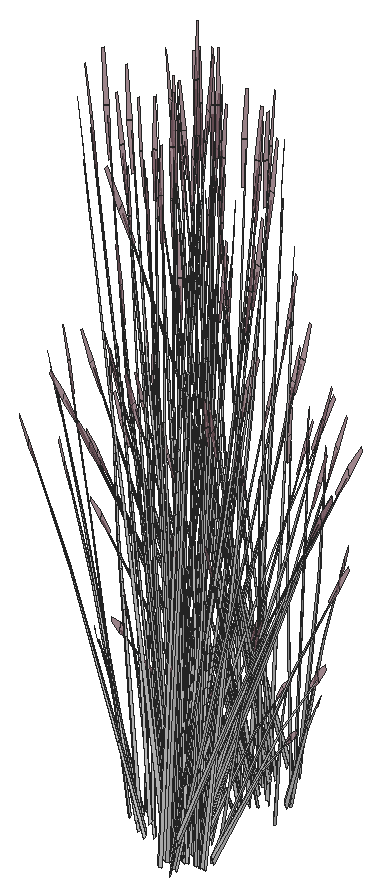
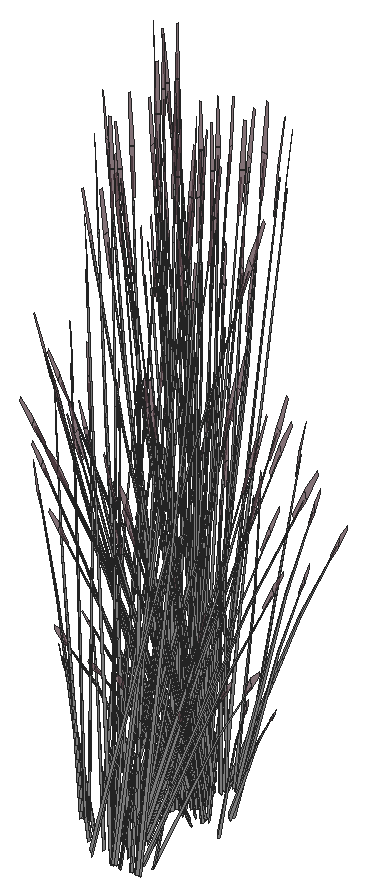
# SketchUp Ruby script. Lengths in inches.
U = 1.inch
M = Sketchup.active_model
def pt(a) = Geom::Point3d.new(a.map { |v| v * U })
def face(e, loops, mat)
  f = e.add_face(loops[0].map { |a| pt(a) })
  loops[1..].each { |l| e.add_face(l.map { |a| pt(a) }).erase! }
  f.material = f.back_material = mat if mat
  f
end
# faces: each face lists its corners as indices into pts; further lists are holes
def faces(e, pts, list, mat = nil) = list.each { |f| face(e, (f[0].is_a?(Array) ? f : [f]).map { |l| l.map { |i| pts[i] } }, mat) }
# xy, xz, yz: faces in a plane at the given z, y or x. An outline is a flat list of corners, or four numbers for a rectangle; further outlines are holes
def ring(l) = l.size == 4 ? [[l[0], l[1]], [l[2], l[1]], [l[2], l[3]], [l[0], l[3]]] : l.each_slice(2).to_a
def flat(e, list, mat, &to3) = list.each { |f| face(e, (f[0].is_a?(Array) ? f : [f]).map { |l| ring(l).map { |u, v| to3.(u, v) } }, mat) }
def xy(e, z, list, mat = nil) = flat(e, list, mat) { |x, y| [x, y, z] }
def xz(e, y, list, mat = nil) = flat(e, list, mat) { |x, z| [x, y, z] }
def yz(e, x, list, mat = nil) = flat(e, list, mat) { |y, z| [x, y, z] }
def lines(e, pts, list) = list.each { |a, b| e.add_line(pt(pts[a]), pt(pts[b])) }
# prism: a flat outline (further loops are holes) pulled along v
def prism(e, loops, v, mat = nil)
  f = face(e, loops, mat); d = Geom::Vector3d.new(v.map { |x| x * U })
  f.pushpull(f.normal.samedirection?(d) ? d.length : -d.length)
end
def box(e, o, s, mat = nil) = prism(e, [[o, [o[0] + s[0], o[1], o[2]], [o[0] + s[0], o[1] + s[1], o[2]], [o[0], o[1] + s[1], o[2]]]], [0, 0, s[2]], mat)
def at(x, y, z, deg = 0) = Geom::Transformation.translation(pt([x, y, z])) * Geom::Transformation.rotation(ORIGIN, Z_AXIS, deg.degrees)
def axes(o, x, y, z) = Geom::Transformation.new([*x, 0, *y, 0, *z, 0, *pt(o).to_a, 1])
def part(name) = M.definitions.add(name)
# library, detail: a bought-in or finely detailed component or shape, given as its bounding box
def library(name, o, s) = part(name).tap { |d| box(d.entities, o, s) }
def detail(e, o, s) = box(e.add_group.entities, o, s)
def put(e, d, t, mat = nil) = e.add_instance(d, t).tap { |i| i.material = mat if mat }
def group(e, t, mat = nil) = e.add_group.tap { |g| g.transformation = t; g.material = mat if mat }.entities
root = M.entities
M.materials.add("LightPink_Translucent").color = [144, 107, 117]
M.materials["LightPink_Translucent"].alpha = 0.75
M.materials.add("[_0053_Ivory_]").color = [200, 200, 200]
c1 = part("blade")
p = [[2.15,0.21,22],[0,0.17,0],[0.09,0.45,0],[2.18,0.31,22],[2.29,0.31,22],[0.38,0.45,0],
  [2.48,0.24,33],[2.49,0.24,33],[2.48,0.22,33]]
faces(c1.entities,p,[[0,1,2,3],[4,5,2,3],[6,3,4,7],[8,0,3,6]])
c2 = part("seeds")
p = [[0.3,-0.1,1.38],[-0.01,-0.03,1.59],[-0.01,-0.03,0.03],[0.14,-0.07,-0.07],[0.29,-0.03,3],[0.15,0.01,3.11]]
faces(c2.entities,p,[[0,1,2,3],[1,0,4,5]],"LightPink_Translucent")
c3 = part("blade with seeds")
put(c3.entities,c1,at(0,0,0))
put(c3.entities,c2,axes([2.4,0.25,30.99],[1.5799,-0.05474,1.17369],[-0.12525,1.92788,0.29478],[-0.07173,-0.02425,1.56792]))
put(root,c3,axes([631.67,325.86,254.32],[-0.61322,0.4175,-0.29095],[-0.40778,-0.58992,-0.50002],[-0.1513,-0.05991,1.59708]),"[_0053_Ivory_]")
put(root,c3,axes([633.01,323.52,254.13],[-0.65264,0.16691,0.17642],[-0.16115,-0.62115,0.35086],[0.05821,0.0905,1.60407]),"[_0053_Ivory_]")
put(root,c3,axes([633.42,324.83,255.53],[-0.25192,0.01424,1.71376],[0.16712,-0.61729,0.13857],[0.35901,0.03818,0.73262]),"[_0053_Ivory_]")
put(root,c3,axes([633.74,323.48,253.68],[0.14267,0.54795,-0.30978],[-0.56663,0.1556,0.30978],[0.11423,0.06319,1.38974]),"[_0053_Ivory_]")
put(root,c3,axes([632.6,324.71,254.03],[-0.76764,-0.13249,0.49198],[0.15622,-0.74829,0.19306],[0.11218,0.07226,1.70813]),"[_0053_Ivory_]")
put(root,c3,axes([631.99,326.56,253.86],[-0.19817,-0.54216,0],[0.56587,-0.18986,0],[0,0,1.54371]),"[_0053_Ivory_]")
put(root,c3,axes([631.61,326.05,254.27],[-0.11717,0.56122,0.1448],[-0.57245,-0.09742,-0.41347],[-0.10418,-0.05763,1.26744]),"[_0053_Ivory_]")
put(root,c3,axes([632.73,326.48,253.84],[0.63764,-0.21337,-0.19198],[0.22406,0.61462,0.00008],[0.07038,-0.02358,1.73897]),"[_0053_Ivory_]")
put(root,c3,axes([632.95,326.74,254.13],[0.17545,-0.62497,0.17642],[0.64204,0.17686,0.35086],[-0.11091,0.00304,1.60407]),"[_0053_Ivory_]")
put(root,c3,axes([632.81,325.32,253.87],[0.42396,0.40619,0],[-0.42396,0.40619,0],[0,0,1.69266]),"[_0053_Ivory_]")
put(root,c3,axes([630.4,324.56,255],[0.17264,-0.09097,1.77064],[0.05953,0.63516,0.13857],[-0.37394,0.08428,0.63284]),"[_0053_Ivory_]")
put(root,c3,axes([633.95,325.15,254.13],[-0.47719,-0.45806,0.17642],[0.48088,-0.44429,0.35086],[-0.0527,0.09355,1.60407]),"[_0053_Ivory_]")
put(root,c3,axes([633.07,324.45,253.71],[0.63179,0.1031,-0.62353],[-0.13332,0.63596,-0.16365],[0.18854,0.07706,1.37633]),"[_0053_Ivory_]")
put(root,c3,axes([635.86,325.56,254.42],[-0.37526,0.10382,1.1486],[0.17664,-0.42906,0.84392],[0.19907,0.02936,0.25299]),"[_0053_Ivory_]")
put(root,c3,axes([631.85,326.8,253.85],[-0.61229,-0.28233,0],[0.29468,-0.58663,0],[0,0,1.62707]),"[_0053_Ivory_]")
put(root,c3,axes([632.36,326.05,254.12],[-0.59306,-0.50614,-0.25192],[0.49904,-0.56836,0.5513],[-0.1597,0.05921,1.68216]),"[_0053_Ivory_]")
put(root,c3,axes([630.8,327.02,254.13],[0.56842,0.31443,0.49651],[-0.33976,0.56381,0],[-0.12946,-0.07161,1.57504]),"[_0053_Ivory_]")
put(root,c3,axes([632.8,324.85,254.37],[0.29468,-0.56664,0.44739],[0.61229,0.27271,-0.21531],[0,0.13062,1.43643]),"[_0053_Ivory_]")
put(root,c3,axes([632.6875,325.17,253.95],[0,0.72727,-0.05637],[-0.75945,0,0],[0,0.02286,1.79368]),"[_0053_Ivory_]")
put(root,c3,axes([629.21,324.91,256.33],[-0.16454,0.57202,-0.51099],[-0.56413,-0.19607,-0.3958],[-0.22713,0.05245,0.97773]),"[_0053_Ivory_]")
put(root,c3,axes([632.74,324.66,253.86],[0.36485,0.52782,-0.44739],[-0.55265,0.37168,0.21531],[0.11807,0.06531,1.43643]),"[_0053_Ivory_]")
put(root,c3,axes([635.21,326.89,255.58],[-0.11624,-0.52862,-0.03492],[0.54943,-0.12153,-0.15832],[0.11473,0.03351,0.52218]),"[_0053_Ivory_]")
put(root,c3,axes([630.47,327.35,254.03],[-0.37973,0.63014,0],[-0.6353,-0.35142,-0.51607],[-0.14469,-0.08004,1.63711]),"[_0053_Ivory_]")
put(root,c3,axes([634.35,325.16,254.13],[0,-0.62885,0.49651],[0.67951,0,0],[0,0.14322,1.57504]),"[_0053_Ivory_]")
put(root,c3,axes([632.65,325.63,254.37],[0.65953,-0.03882,0.44739],[0.05964,0.64439,-0.21531],[-0.11807,0.06531,1.43643]),"[_0053_Ivory_]")
put(root,c3,axes([633.06,324.98,254.27],[0.56587,-0.18339,0.1448],[0.19817,0.52368,-0.41347],[0,0.11525,1.26744]),"[_0053_Ivory_]")
put(root,c3,axes([632.06,325.95,253.86],[-0.65953,0.03882,-0.44739],[-0.05964,-0.64439,0.21531],[-0.11807,0.06531,1.43643]),"[_0053_Ivory_]")
put(root,c3,axes([635.16,326.25,254.24],[-0.14627,-0.15466,1.43002],[0.19032,-0.51164,-0.30754],[0.29594,0.06931,0.61141]),"[_0053_Ivory_]")
put(root,c3,axes([632.55,326.82,253.86],[0.61229,0.28233,0],[-0.29468,0.58663,0],[0,0,1.74954]),"[_0053_Ivory_]")
put(root,c3,axes([632.79,327.44,253.85],[-0.37499,-0.63235,-0.05142],[0.6353,-0.35142,0.51607],[-0.15655,0.0602,1.6363]),"[_0053_Ivory_]")
put(root,c3,axes([632.66,325.91,254.27],[0.44871,0.37783,0.1448],[-0.37428,0.42627,-0.41347],[-0.10418,0.05763,1.26744]),"[_0053_Ivory_]")
put(root,c3,axes([629.1875,325.2,255.53],[0.21074,-0.13302,1.71376],[0.17741,0.61464,0.13857],[-0.33083,0.13891,0.73262]),"[_0053_Ivory_]")
put(root,c3,axes([633.82,326.5625,256.63],[0.60713,0.01514,-0.71045],[-0.04078,0.63759,0.08574],[0.25721,0.06729,1.00501]),"[_0053_Ivory_]")
put(root,c3,axes([633.13,327.08,254.13],[0.56842,-0.31443,0.49651],[0.33976,0.56381,0],[-0.12946,0.07161,1.57504]),"[_0053_Ivory_]")
put(root,c3,axes([632.32,326.58,253.94],[0.26406,0.72244,-0.06012],[-0.7545,0.25315,0],[0.00922,0.02523,1.72173]),"[_0053_Ivory_]")
put(root,c3,axes([632.62,327.36,253.68],[-0.56663,-0.1556,-0.30978],[0.14267,-0.54795,0.30978],[-0.11423,0.06319,1.38974]),"[_0053_Ivory_]")
put(root,c3,axes([628.53,326.25,254.24],[0.21107,0.05162,1.43002],[0.13604,0.52729,-0.30754],[-0.28671,0.0987,0.61141]),"[_0053_Ivory_]")
put(root,c3,axes([634.81,325.27,254.03],[0.75945,0,0],[0,0.70283,-0.51607],[0,0.16007,1.63711]),"[_0053_Ivory_]")
put(root,c3,axes([634.51,325.63,253.85],[-0.75908,-0.00503,-0.04976],[0,-0.70283,0.49943],[-0.02386,0.16,1.58352]),"[_0053_Ivory_]")
put(root,c3,axes([632.86,325.02,254.32],[0.68399,0.30005,-0.29095],[-0.32934,0.63331,-0.50002],[0.0215,0.15549,1.59708]),"[_0053_Ivory_]")
put(root,c3,axes([628.09,327.35,254.42],[0.25312,-0.28501,1.1486],[0.09988,0.45119,0.84392],[-0.18292,0.08079,0.25299]),"[_0053_Ivory_]")
put(root,c3,axes([634.18,326.83,256.18],[0.34557,0.39372,-0.35414],[-0.39459,0.37271,0.4572],[0.20048,0.05671,0.87481]),"[_0053_Ivory_]")
put(root,c3,axes([634.35,325.73,253.68],[-0.42396,0.39235,-0.30978],[-0.42396,-0.39235,0.30978],[0,0.12637,1.38974]),"[_0053_Ivory_]")
put(root,c3,axes([632.52,325.77,254.32],[0.07077,0.71755,-0.29095],[-0.73712,0.04339,-0.50002],[-0.1298,0.09558,1.59708]),"[_0053_Ivory_]")
put(root,c3,axes([632.79,325.49,253.86],[-0.29468,0.56664,-0.44739],[-0.61229,-0.27271,0.21531],[0,0.13062,1.43643]),"[_0053_Ivory_]")
put(root,c3,axes([629.04,326.12,256.18],[-0.52868,0.08987,-0.35414],[-0.1396,-0.51376,0.4572],[-0.1515,0.13799,0.87481]),"[_0053_Ivory_]")
put(root,c3,axes([630.49,334.45,255.53],[0.13883,0.2019,1.71376],[-0.64153,0.16998,0.13857],[-0.14499,-0.31697,0.73262]),"[_0053_Ivory_]")
put(root,c3,axes([632.08,326.32,253.71],[-0.40909,0.47266,-0.62353],[-0.50819,-0.4286,-0.16365],[-0.16393,0.11791,1.37633]),"[_0053_Ivory_]")
put(root,c3,axes([632.81,327.12,253.98],[0.76036,0.2044,0.30756],[-0.19023,0.7306,-0.36492],[-0.12585,0.09144,1.64885]),"[_0053_Ivory_]")
put(root,c3,axes([632.75,327.61,253.67],[-0.56842,0.31443,-0.49651],[-0.33976,-0.56381,0],[-0.12946,0.07161,1.57504]),"[_0053_Ivory_]")
put(root,c3,axes([634.64,325.75,253.67],[0,0.62885,-0.49651],[-0.67951,0,0],[0,0.14322,1.57504]),"[_0053_Ivory_]")
put(root,c3,axes([632.94,325.82,255.53],[-0.2256,-0.10835,1.71376],[0.46687,-0.45453,0.13857],[0.29098,0.20505,0.73262]),"[_0053_Ivory_]")
put(root,c3,axes([632.98,334.16,254.24],[-0.17264,0.12729,1.43002],[-0.51703,-0.22279,-0.30754],[0.09584,-0.27707,0.61141]),"[_0053_Ivory_]")
put(root,c3,axes([632.2,334.6,256.63],[-0.28988,-0.51132,-0.71045],[0.59671,-0.28496,0.08574],[-0.06778,-0.24706,1.00501]),"[_0053_Ivory_]")
put(root,c3,axes([630.3125,333.92,254.24],[-0.03678,0.20572,1.43002],[-0.53767,0.17221,-0.30754],[-0.12568,-0.26589,0.61141]),"[_0053_Ivory_]")
put(root,c3,axes([633.78,327.05,254.42],[-0.34197,-0.18082,1.1486],[0.44156,-0.18372,0.84392],[0.1191,0.15563,0.25299]),"[_0053_Ivory_]")
put(root,c3,axes([631.7,333.47,253.15],[-0.10187,0.02266,1.76342],[-0.56336,-0.25503,-0.26939],[0.00945,-0.21273,0.30037]),"[_0053_Ivory_]")
put(root,c3,axes([629.96,325.62,255.53],[0.1517,-0.19322,1.71376],[0.38303,0.52154,0.13857],[-0.26271,0.23751,0.73262]),"[_0053_Ivory_]")
put(root,c3,axes([633.4,335.1,256.63],[0.0158,-0.58168,-0.71045],[0.66548,0.03907,0.08574],[0.07023,-0.24643,1.00501]),"[_0053_Ivory_]")
put(root,c3,axes([629.48,326.18,256.33],[0.15602,0.5742,-0.51099],[-0.59087,0.10045,-0.3958],[-0.16933,0.15423,0.97773]),"[_0053_Ivory_]")
put(root,c3,axes([633.27,327.51,254.03],[0.37973,0.63014,0],[-0.6353,0.35142,-0.51607],[-0.14469,0.08004,1.63711]),"[_0053_Ivory_]")
put(root,c3,axes([632.25,334.17,256.18],[0.1831,-0.48359,-0.35414],[0.53419,0.14105,0.4572],[-0.04898,-0.1947,0.87481]),"[_0053_Ivory_]")
put(root,c3,axes([632.65,334.81,255.53],[-0.11309,0.21615,1.71376],[-0.47441,-0.44731,0.13857],[0.21402,-0.27879,0.73262]),"[_0053_Ivory_]")
put(root,c3,axes([633.87,327.72,253.15],[0.04425,-0.09079,1.76342],[0.55709,-0.26738,-0.26939],[0.16889,0.13839,0.30037]),"[_0053_Ivory_]")
put(root,c3,axes([632.94,325.02,254.5],[-0.01659,-0.59209,1.41272],[0.75089,0.15348,0.59816],[-0.1776,0.32398,1.3335]),"[_0053_Ivory_]")
put(root,c3,axes([633.14,325.66,253.75],[0.2227,0.57576,-0.69212],[-0.64151,0.20736,-0.18165],[0.02462,0.19497,1.52773]),"[_0053_Ivory_]")
put(root,c3,axes([628.76,327.65,253.15],[0.08147,0.06283,1.76342],[0.13814,0.58211,-0.26939],[-0.18056,0.12413,0.30037]),"[_0053_Ivory_]")
put(root,c3,axes([633,327.3,256.33],[0.59932,-0.14948,-0.51099],[0.10484,0.56611,-0.3958],[0.16097,0.16223,0.97773]),"[_0053_Ivory_]")
put(root,c3,axes([631.98,334.5,256.33],[-0.59704,-0.15764,-0.51099],[0.20464,-0.54049,-0.3958],[-0.05475,-0.21761,0.97773]),"[_0053_Ivory_]")
put(root,c3,axes([632.35,333.15,254.42],[0.07791,0.3667,1.1486],[-0.43222,-0.2031,0.84392],[0.04651,-0.18776,0.25299]),"[_0053_Ivory_]")
put(root,c3,axes([633.27,334.91,256.33],[-0.43478,-0.42253,-0.51099],[0.45929,-0.37004,-0.3958],[0.06615,-0.21468,0.97773]),"[_0053_Ivory_]")
put(root,c3,axes([633.83,327.875,254.32],[-0.38947,-0.01972,1.0506],[0.25721,-0.41888,0.58006],[0.15386,0.14882,0.8241]),"[_0053_Ivory_]")
put(root,c3,axes([633.68,334.75,256.18],[0.41095,-0.33109,-0.35414],[0.38901,0.37805,0.4572],[0.05919,-0.19208,0.87481]),"[_0053_Ivory_]")
put(root,c3,axes([630.125,333.59,254.42],[0.31682,0.21887,1.1486],[-0.4614,0.13157,0.84392],[-0.09872,-0.16821,0.25299]),"[_0053_Ivory_]")
put(root,c3,axes([630.89,334.75,256.63],[-0.51789,-0.30395,-0.71045],[0.36805,-0.53263,0.08574],[-0.18764,-0.18149,1.00501]),"[_0053_Ivory_]")
put(root,c3,axes([629.84,326.09,255.53],[0.11309,-0.21615,1.71376],[0.47441,0.44731,0.13857],[-0.21402,0.27879,0.73262]),"[_0053_Ivory_]")
put(root,c3,axes([630.71,334.35,256.18],[-0.0938,-0.50652,-0.35414],[0.53623,-0.13375,0.4572],[-0.14403,-0.14515,0.87481]),"[_0053_Ivory_]")
put(root,c3,axes([632.56,326.86,254.24],[0.01072,-0.20846,1.43002],[0.51218,-0.23285,-0.30754],[0.15811,0.2495,0.61141]),"[_0053_Ivory_]")
put(root,c3,axes([629.97,327.31,256.18],[-0.41095,0.33109,-0.35414],[-0.38901,-0.37805,0.4572],[-0.05919,0.19208,0.87481]),"[_0053_Ivory_]")
put(root,c3,axes([630.24,328.6,254.42],[-0.01572,-0.37392,1.1486],[0.39276,0.26669,0.84392],[-0.07724,0.17822,0.25299]),"[_0053_Ivory_]")
put(root,c3,axes([629.875,334.25,253.15],[-0.05883,0.08284,1.76342],[-0.59454,0.17861,-0.26939],[-0.14363,-0.16248,0.30037]),"[_0053_Ivory_]")
put(root,c3,axes([631.27,327.7,253.15],[0.09829,-0.03422,1.76342],[0.59126,0.18834,-0.26939],[0.01729,0.21228,0.30037]),"[_0053_Ivory_]")
put(root,c3,axes([630.86,336.52,253.75],[-0.24943,-0.64486,-0.69835],[0.71849,-0.23224,-0.18329],[-0.02757,-0.21836,1.54149]),"[_0053_Ivory_]")
put(root,c3,axes([629.56,335.08,255.53],[0.2256,0.10835,1.71376],[-0.46687,0.45453,0.13857],[-0.29098,-0.20505,0.73262]),"[_0053_Ivory_]")
put(root,c3,axes([634.19,334.55,253.15],[-0.0909,-0.04954,1.76342],[-0.2335,-0.55347,-0.26939],[0.15752,-0.1502,0.30037]),"[_0053_Ivory_]")
put(root,c3,axes([630.38,327.15,256.66],[0.43478,0.42253,-0.5672],[-0.45929,0.37004,-0.43934],[-0.06615,0.21468,1.08528]),"[_0053_Ivory_]")
put(root,c3,axes([629.91,327.79,254.48],[0.55175,-0.11136,0.06507],[0.12684,0.44864,-0.86304],[-0.03498,0.22711,0.7736]),"[_0053_Ivory_]")
put(root,c3,axes([631.67,327.5625,256.33],[0.59704,0.15764,-0.51099],[-0.20464,0.54049,-0.3958],[0.05475,0.21761,0.97773]),"[_0053_Ivory_]")
put(root,c3,axes([632.01,326.45,255.53],[-0.13883,-0.2019,1.71376],[0.64153,-0.16998,0.13857],[0.14499,0.31697,0.73262]),"[_0053_Ivory_]")
put(root,c3,axes([630.65,334.76,256.33],[-0.59932,0.14948,-0.51099],[-0.10484,-0.56611,-0.3958],[-0.16097,-0.16223,0.97773]),"[_0053_Ivory_]")
put(root,c3,axes([631.4,327.9,256.18],[-0.1831,0.48359,-0.35414],[-0.53419,-0.14105,0.4572],[0.04898,0.1947,0.87481]),"[_0053_Ivory_]")
put(root,c3,axes([634.1875,336.12,256.63],[0.31725,-0.49618,-0.71045],[0.55593,0.35263,0.08574],[0.18942,-0.17977,1.00501]),"[_0053_Ivory_]")
put(root,c3,axes([630.76,334.67,254.03],[-0.37973,-0.63014,0],[0.6353,-0.35142,-0.51607],[0.14469,-0.08004,1.63711]),"[_0053_Ivory_]")
put(root,c3,axes([634.17,335.88,256.33],[-0.15602,-0.5742,-0.51099],[0.59087,-0.10045,-0.3958],[0.16933,-0.15423,0.97773]),"[_0053_Ivory_]")
put(root,c3,axes([630.25,326.96,256.99],[-0.0158,0.58168,-0.7886],[-0.66548,-0.03907,0.09517],[-0.07023,0.24643,1.11556]),"[_0053_Ivory_]")
put(root,c3,axes([631.59,333.91,253.78],[-0.4197,0.36076,-0.03893],[-0.38456,-0.39511,-0.17649],[-0.02707,-0.11196,0.58215]),"[_0053_Ivory_]")
put(root,c3,axes([630.88,326.55,255.53],[-0.01487,-0.24136,1.71376],[0.64429,0.16012,0.13857],[-0.03985,0.34396,0.73262]),"[_0053_Ivory_]")
put(root,c3,axes([631.46,327.46,256.63],[0.28988,0.51132,-0.71045],[-0.59671,0.28496,0.08574],[0.06778,0.24706,1.00501]),"[_0053_Ivory_]")
put(root,c3,axes([632.13,338.1875,254.98],[0.52485,0.25358,1.51261],[-0.51417,0.54629,0.59816],[-0.23031,-0.32378,1.26806]),"[_0053_Ivory_]")
put(root,c3,axes([629.78,328.26,254.24],[0.19166,-0.0992,1.43002],[0.4732,0.29912,-0.30754],[-0.14084,0.25882,0.61141]),"[_0053_Ivory_]")
put(root,c3,axes([629.39,336.43,253.67],[0,-0.62885,-0.49651],[0.67951,0,0],[0,-0.14322,1.57504]),"[_0053_Ivory_]")
put(root,c3,axes([631.27,334.57,253.67],[0.56842,-0.31443,-0.49651],[0.33976,0.56381,0],[0.12946,-0.07161,1.57504]),"[_0053_Ivory_]")
put(root,c3,axes([634.65,335.66,254.24],[-0.21697,-0.01863,1.43002],[-0.22228,-0.49966,-0.30754],[0.26655,-0.14135,0.61141]),"[_0053_Ivory_]")
put(root,c3,axes([631.95,335.86,253.71],[0.40909,-0.47266,-0.62353],[0.50819,0.4286,-0.16365],[0.16393,-0.11791,1.37633]),"[_0053_Ivory_]")
put(root,c3,axes([634.9,334.74,254.42],[-0.2023,0.32011,1.1486],[-0.17388,-0.43009,0.84392],[0.16708,-0.10777,0.25299]),"[_0053_Ivory_]")
put(root,c3,axes([634.61,335.94,256.18],[0.52868,-0.08987,-0.35414],[0.1396,0.51376,0.4572],[0.1515,-0.13799,0.87481]),"[_0053_Ivory_]")
put(root,c3,axes([631.24,336.69,253.86],[0.29468,-0.56664,-0.44739],[0.61229,0.27271,0.21531],[0,-0.13062,1.43643]),"[_0053_Ivory_]")
put(root,c3,axes([629.47,335.24,256.18],[-0.34557,-0.39372,-0.35414],[0.39459,-0.37271,0.4572],[-0.20048,-0.05671,0.87481]),"[_0053_Ivory_]")
put(root,c3,axes([630.03,327.78,255.02],[0.01334,-0.32463,1.54345],[0.60018,0.17147,0.21329],[-0.052,0.34598,0.72882]),"[_0053_Ivory_]")
put(root,c3,axes([631.5,336.41,254.32],[-0.07077,-0.71755,-0.29095],[0.73712,-0.04339,-0.50002],[0.1298,-0.09558,1.59708]),"[_0053_Ivory_]")
put(root,c3,axes([629.68,336.45,253.68],[0.42396,-0.39235,-0.30978],[0.42396,0.39235,0.30978],[0,-0.12637,1.38974]),"[_0053_Ivory_]")
put(root,c3,axes([629.51,334.57,253.78],[-0.1752,0.51349,-0.03893],[-0.53924,-0.15795,-0.17649],[-0.08187,-0.08399,0.58215]),"[_0053_Ivory_]")
put(root,c3,axes([631.16,337.16,254.32],[-0.68399,-0.30005,-0.29095],[0.32934,-0.63331,-0.50002],[-0.0215,-0.15549,1.59708]),"[_0053_Ivory_]")
put(root,c3,axes([629.22,336.91,254.03],[-0.75945,0,0],[0,-0.70283,-0.51607],[0,-0.16007,1.63711]),"[_0053_Ivory_]")
put(root,c3,axes([629.35,335.66,254.24],[0.11858,0.17508,1.43002],[-0.27325,0.4759,-0.30754],[-0.28057,-0.11375,0.61141]),"[_0053_Ivory_]")
